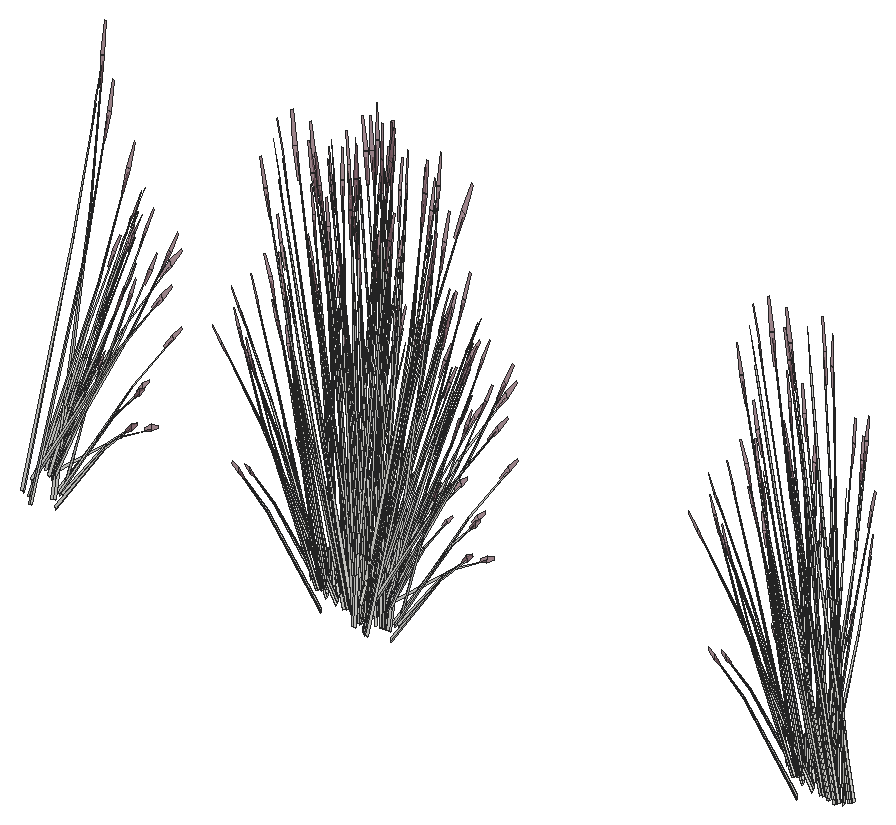
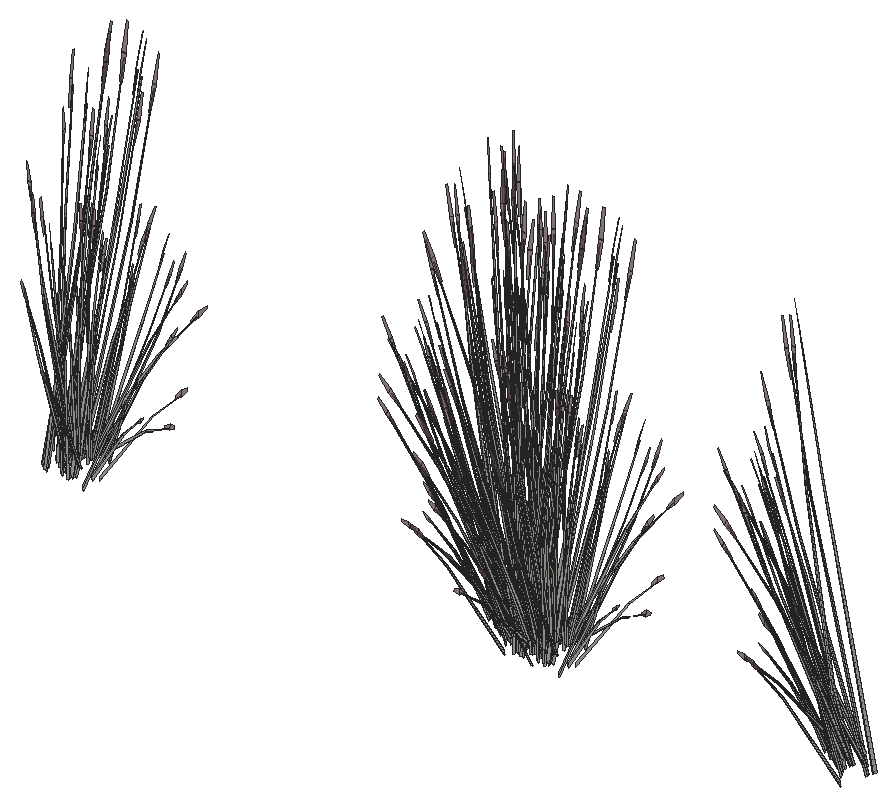
# SketchUp Ruby script. Lengths in inches.
U = 1.inch
M = Sketchup.active_model
def pt(a) = Geom::Point3d.new(a.map { |v| v * U })
def face(e, loops, mat)
  f = e.add_face(loops[0].map { |a| pt(a) })
  loops[1..].each { |l| e.add_face(l.map { |a| pt(a) }).erase! }
  f.material = f.back_material = mat if mat
  f
end
# faces: each face lists its corners as indices into pts; further lists are holes
def faces(e, pts, list, mat = nil) = list.each { |f| face(e, (f[0].is_a?(Array) ? f : [f]).map { |l| l.map { |i| pts[i] } }, mat) }
# xy, xz, yz: faces in a plane at the given z, y or x. An outline is a flat list of corners, or four numbers for a rectangle; further outlines are holes
def ring(l) = l.size == 4 ? [[l[0], l[1]], [l[2], l[1]], [l[2], l[3]], [l[0], l[3]]] : l.each_slice(2).to_a
def flat(e, list, mat, &to3) = list.each { |f| face(e, (f[0].is_a?(Array) ? f : [f]).map { |l| ring(l).map { |u, v| to3.(u, v) } }, mat) }
def xy(e, z, list, mat = nil) = flat(e, list, mat) { |x, y| [x, y, z] }
def xz(e, y, list, mat = nil) = flat(e, list, mat) { |x, z| [x, y, z] }
def yz(e, x, list, mat = nil) = flat(e, list, mat) { |y, z| [x, y, z] }
def lines(e, pts, list) = list.each { |a, b| e.add_line(pt(pts[a]), pt(pts[b])) }
# prism: a flat outline (further loops are holes) pulled along v
def prism(e, loops, v, mat = nil)
  f = face(e, loops, mat); d = Geom::Vector3d.new(v.map { |x| x * U })
  f.pushpull(f.normal.samedirection?(d) ? d.length : -d.length)
end
def box(e, o, s, mat = nil) = prism(e, [[o, [o[0] + s[0], o[1], o[2]], [o[0] + s[0], o[1] + s[1], o[2]], [o[0], o[1] + s[1], o[2]]]], [0, 0, s[2]], mat)
def at(x, y, z, deg = 0) = Geom::Transformation.translation(pt([x, y, z])) * Geom::Transformation.rotation(ORIGIN, Z_AXIS, deg.degrees)
def axes(o, x, y, z) = Geom::Transformation.new([*x, 0, *y, 0, *z, 0, *pt(o).to_a, 1])
def part(name) = M.definitions.add(name)
# library, detail: a bought-in or finely detailed component or shape, given as its bounding box
def library(name, o, s) = part(name).tap { |d| box(d.entities, o, s) }
def detail(e, o, s) = box(e.add_group.entities, o, s)
def put(e, d, t, mat = nil) = e.add_instance(d, t).tap { |i| i.material = mat if mat }
def group(e, t, mat = nil) = e.add_group.tap { |g| g.transformation = t; g.material = mat if mat }.entities
root = M.entities
M.materials.add("LightPink_Translucent").color = [144, 107, 117]
M.materials["LightPink_Translucent"].alpha = 0.75
c1 = part("blade")
p = [[2.15,0.21,22],[0,0.17,0],[0.09,0.45,0],[2.18,0.31,22],[2.29,0.31,22],[0.38,0.45,0],
  [2.48,0.24,33],[2.49,0.24,33],[2.48,0.22,33]]
faces(c1.entities,p,[[0,1,2,3],[4,5,2,3],[6,3,4,7],[8,0,3,6]])
c2 = part("seeds")
p = [[0.3,-0.1,1.38],[-0.01,-0.03,1.59],[-0.01,-0.03,0.03],[0.14,-0.07,-0.07],[0.29,-0.03,3],[0.15,0.01,3.11]]
faces(c2.entities,p,[[0,1,2,3],[1,0,4,5]],"LightPink_Translucent")
c3 = part("blade with seeds")
put(c3.entities,c1,at(0,0,0))
put(c3.entities,c2,axes([2.4,0.25,30.99],[1.5799,-0.05474,1.17369],[-0.12525,1.92788,0.29478],[-0.07173,-0.02425,1.56792]))
put(root,c3,axes([763.12,481.41,3.1875],[0.57465,0,0],[0,0.36542,-0.25804],[0,0.08323,0.81856]))
put(root,c3,axes([761.26,480.94,3.33],[0.46399,-0.21707,-0.14548],[0.30855,0.30672,-0.25001],[0.11448,0.03115,0.79854]))
put(root,c3,axes([762.375,482.77,3.33],[-0.2947,-0.01025,0.5253],[0.19462,-0.21779,0.29003],[0.11642,0.07737,0.41205]))
put(root,c3,axes([761.43,482.61,4.52],[0.27385,-0.27986,-0.0608],[0.39658,0.16123,-0.33747],[0.13785,0.07907,0.51278]))
put(root,c3,axes([761.75,482.47,4.34],[0.45348,-0.07772,-0.25549],[0.07933,0.29434,-0.1979],[0.1218,0.08435,0.48886]))
put(root,c3,axes([762.27,482.12,4.53],[-0.26148,-0.20471,0.17707],[0.29857,-0.19378,-0.2286],[0.1517,0.02948,0.4374]))
put(root,c3,axes([762.43,480.36,3.01],[0.4301,0.16348,-0.24825],[-0.25708,0.29314,0],[0.09796,0.03723,0.78752]))
put(root,c3,axes([762.51,482.3,4.37],[-0.02314,0.24862,0.03215],[-0.34943,-0.00682,0.2531],[0.13385,0.02602,0.38595]))
put(root,c3,axes([762.41,482.69,2.75],[0.03348,-0.0472,0.88171],[0.42153,-0.13902,-0.1347],[0.12779,0.07195,0.15018]))
put(root,c3,axes([762.54,482.22,4.37],[-0.33886,0.21544,0.24001],[-0.29224,-0.22879,0.1979],[0.15898,0.03974,0.49665]))
put(root,c3,axes([763.42,482.26,3.96],[-0.08796,-0.27485,-0.01746],[0.41573,-0.06319,-0.07916],[0.08682,0.01742,0.26109]))
put(root,c3,axes([761.8,480.99,3.03],[0.47805,0.0536,-0.31177],[-0.10088,0.33065,-0.08182],[0.14266,0.04007,0.68817]))
put(root,c3,axes([761.7,481.7,3.9375],[-0.1707,-0.05633,0.85688],[0.35326,-0.23632,0.06928],[0.22018,0.10661,0.36631]))
put(root,c3,axes([763.05,481.625,4.37],[0.16879,0.22293,0.03215],[-0.30779,0.10912,0.2531],[0.13568,-0.02153,0.38595]))
put(root,c3,axes([762.64,482.22,4.26],[0.26148,0.20471,-0.17707],[-0.29857,0.19378,0.2286],[0.1517,0.02948,0.4374]))
put(root,c3,axes([762.34,482.25,4.52],[0.02461,-0.33251,-0.0608],[0.4659,0.00909,-0.33747],[0.17944,0.0231,0.51278]))
put(root,c3,axes([763.01,481.55,4.37],[-0.12984,0.29812,0.24001],[-0.42685,-0.10194,0.1979],[0.16786,-0.01792,0.49665]))
put(root,c3,axes([762.75,482.05,4.36],[0.09858,-0.00553,0.87472],[0.2704,-0.25401,-0.13834],[0.17535,0.03353,0.07015]))
put(root,c3,axes([763.91,481.57,3.38],[-0.28394,0.05398,0.5743],[0.13365,-0.22308,0.42196],[0.15063,0.01526,0.12649]))
put(root,c3,axes([763.1,481.51,4.26],[0.38192,0.09121,-0.17707],[-0.11139,0.2661,0.2286],[0.15377,-0.0244,0.4374]))
put(root,c3,axes([762.37,482.09,4.49],[0.45939,0.00787,-0.35523],[-0.03085,0.3315,0.04287],[0.19462,0.03498,0.5025]))
put(root,c3,axes([763.62,481.26,2.75],[-0.02402,-0.04964,0.88171],[0.16658,-0.29036,-0.1347],[0.16804,-0.00418,0.15018]))
put(root,c3,axes([763.78,482.51,4.35],[-0.04155,-0.02862,0.88692],[0.0909,-0.30682,-0.08381],[0.16368,-0.0196,0.15695]))
put(root,c3,axes([762.0625,481.18,3.9375],[-0.19062,0.00741,0.85688],[0.12645,-0.32094,0.06928],[0.27165,0.01985,0.36631]))
put(root,c3,axes([763.38,481.93,3.3],[-0.11068,-0.08041,0.71501],[0.144,-0.26601,-0.15377],[0.22393,0.03604,0.3057]))
put(root,c3,axes([782.62,481.38,3.9375],[0.15946,-0.06916,0.85688],[0.13424,0.31957,0.06928],[-0.25033,0.07223,0.36631]))
put(root,c3,axes([782.125,481.92,3.3],[0.15971,0.02684,0.71501],[0.10294,0.27415,-0.15377],[-0.21694,0.05132,0.3057]))
put(root,c3,axes([783.54,481.05,3.67],[0.13063,-0.0473,0.88532],[0.04505,0.33024,0.06928],[-0.28294,0.04382,0.31642]))
put(root,c3,axes([782.13,481.27,4.36],[-0.07505,0.04245,0.87472],[0.00638,0.31015,-0.13834],[-0.17202,0.04033,0.07015]))
put(root,c3,axes([782.375,481.09,4.26],[-0.38192,-0.09121,-0.17707],[0.11139,-0.2661,0.2286],[-0.15377,0.0244,0.4374]))
put(root,c3,axes([781.3,481.58,4.35],[0.05865,0.00877,0.88692],[0.18143,0.28888,-0.08381],[-0.12006,0.07582,0.15695]))
put(root,c3,axes([782.64,481.23,4.34],[-0.1245,0.29741,-0.25549],[-0.42685,-0.10194,-0.1979],[-0.17186,0.02727,0.48886]))
put(root,c3,axes([782.42,481.21,2.75],[0.01165,0.05153,0.88171],[-0.23495,0.26909,-0.1347],[-0.16689,-0.01356,0.15018]))
put(root,c3,axes([781.79,482.5,3.38],[0.19152,-0.14818,0.5743],[0.07557,0.23459,0.42196],[-0.13841,0.042,0.12649]))
put(root,c3,axes([782.62,480.97,4.52],[0.23123,0.29606,-0.0608],[-0.41039,0.14549,-0.33747],[-0.17294,0.03906,0.51278]))
put(root,c3,axes([782.43,480.98,4.37],[-0.16879,-0.22293,0.03215],[0.30779,-0.10912,0.2531],[-0.13568,0.02153,0.38595]))
put(root,c3,axes([783.21,481.59,3.9375],[0.11478,-0.10046,0.85688],[0.28982,0.27117,0.06928],[-0.19878,0.12349,0.36631]))
put(root,c3,axes([782.52,481.86,4.26],[-0.40003,0.04673,-0.17707],[-0.10563,-0.26712,0.2286],[-0.11464,0.07175,0.4374]))
put(root,c3,axes([782.3,482.65,2.75],[0.06164,0.03267,0.88171],[0.10452,0.30266,-0.1347],[-0.13662,0.06454,0.15018]))
put(root,c3,axes([782.57,481.8,4.37],[-0.11397,-0.30091,0.24001],[0.44709,-0.05222,0.1979],[-0.13177,0.07077,0.49665]))
put(root,c3,axes([782.48,481.74,4.37],[-0.31549,-0.13751,0.03215],[0.18368,-0.19581,0.2531],[-0.10115,0.06331,0.38595]))
put(root,c3,axes([783.12,481.84,3.9375],[0.08557,-0.11238,0.85688],[0.35897,0.23257,0.06928],[-0.16194,0.14495,0.36631]))
put(root,c3,axes([782.78,481.06,4.53],[0.38192,0.09121,0.17707],[-0.11139,0.2661,-0.2286],[-0.15377,0.0244,0.4374]))
put(root,c3,axes([782.85,481.89,4.34],[0.11806,0.29854,-0.25549],[-0.44709,0.05222,-0.1979],[-0.12812,0.08019,0.48886]))
put(root,c3,axes([782.15,482.42,4.36],[-0.01142,0.0647,0.87472],[0.32418,0.22509,-0.13834],[-0.08487,0.10644,0.07015]))
put(root,c3,axes([783.33,482.3,3.01],[-0.4301,-0.16348,-0.24825],[0.25708,-0.29314,0],[-0.09796,-0.03723,0.78752]))
put(root,c3,axes([782.63,481.67,4.52],[0.4251,0.18028,-0.0608],[-0.24491,0.26108,-0.33747],[-0.1201,0.09075,0.51278]))
put(root,c3,axes([783.59,482.5,3.1875],[-0.28732,0.32763,0],[-0.4807,-0.18271,-0.25804],[-0.10948,-0.04161,0.81856]))
put(root,c3,axes([781.93,482.46,4.82],[0.40553,0.08728,-0.03244],[-0.12475,0.26862,-0.14708],[-0.06633,0.04078,0.48512]))
put(root,c3,axes([782.84,481.7,4.53],[0.40003,-0.04673,0.17707],[0.10563,0.26712,-0.2286],[-0.11464,0.07175,0.4374]))
put(root,c3,axes([783.07,482.97,3.3],[0.14502,-0.05158,0.71501],[0.35805,0.15552,-0.15377],[-0.10657,0.13457,0.3057]))
put(root,c3,axes([784.5,481.72,3.33],[-0.46399,0.21707,-0.14548],[-0.30855,-0.30672,-0.25001],[-0.11448,-0.03115,0.79854]))
put(root,c3,axes([783.22,482.41,4.37],[-0.32725,-0.22308,0.24001],[0.34753,-0.1924,0.1979],[-0.06036,0.10466,0.49665]))
put(root,c3,axes([783.45,482.18,3.01],[-0.10795,-0.28489,-0.15489],[0.42874,-0.0809,0.15489],[-0.08643,-0.03285,0.69487]))
put(root,c3,axes([783.1,482.39,4.37],[-0.37765,-0.01523,0.03215],[0.01035,-0.23004,0.2531],[-0.03952,0.08812,0.38595]))
put(root,c3,axes([783.22,482.48,4.26],[-0.31095,0.17214,-0.17707],[-0.29435,-0.19656,0.2286],[-0.04479,0.09987,0.4374]))
put(root,c3,axes([784.8125,481.96,3.03],[-0.30954,0.24575,-0.31177],[-0.38452,-0.22284,-0.08182],[-0.12404,0.0613,0.68817]))
put(root,c3,axes([782.11,483.09,4.35],[0.05214,-0.01974,0.88692],[0.43092,0.1313,-0.08381],[-0.01013,0.10932,0.15695]))
put(root,c3,axes([785.02,481.82,3.23],[-0.44875,-0.26316,-0.12596],[0.3776,-0.2955,0.27565],[-0.12084,0.03078,0.84108]))
put(root,c3,axes([783.43,482.29,4.67],[-0.01196,0.30243,-0.3943],[-0.50354,-0.02031,0.04758],[-0.05314,0.12813,0.55778]))
put(root,c3,axes([783.42,483.14,3.38],[-0.01189,-0.19441,0.5743],[0.29719,0.13866,0.42196],[-0.05845,0.09266,0.12649]))
put(root,c3,axes([784.8,481.77,3.11],[-0.49904,0.02018,-0.2237],[-0.04513,-0.33504,0.10766],[-0.08934,0.03396,0.71822]))
put(root,c3,axes([783.84,482.33,3.24],[0.4301,0.16348,0.24825],[-0.25708,0.29314,0],[-0.09796,-0.03723,0.78752]))
put(root,c3,axes([783.26,482.72,3.68],[0.0101,-0.16879,0.77173],[0.45413,0.08915,0.10664],[-0.03935,0.17989,0.36441]))
put(root,c3,axes([784.46,481.82,3.31],[-0.08866,0.29179,0.0724],[-0.43315,-0.05065,-0.20674],[-0.07883,-0.02996,0.63372]))
put(root,c3,axes([785.32,482.63,3.01],[-0.4301,0.16348,-0.24825],[-0.25708,-0.29314,0],[-0.09796,0.03723,0.78752]))
put(root,c3,axes([785.35,482.54,3.1],[-0.28374,-0.32877,-0.02571],[0.4807,-0.18271,0.25804],[-0.11845,0.0313,0.81815]))
put(root,c3,axes([783.53,482.39,4.5],[0.32898,0.21969,-0.2836],[-0.34753,0.1924,-0.21967],[-0.05006,0.11162,0.54264]))
put(root,c3,axes([785.22,482.5,3.01],[-0.42874,-0.0809,-0.15489],[0.10795,-0.28489,0.15489],[-0.08643,0.03285,0.69487]))
put(root,c3,axes([783.38,482.23,4.53],[0.31095,-0.17214,0.17707],[0.29435,0.19656,-0.2286],[-0.04479,0.09987,0.4374]))
put(root,c3,axes([785.47,481.28,3.42],[-0.01255,-0.30784,0.70636],[0.56816,0.0798,0.29908],[-0.13438,0.16845,0.66675]))
put(root,c3,axes([783.18,482.28,4.7],[0.50507,0.0162,-0.06749],[-0.01381,0.30672,-0.3746],[-0.03508,0.11813,0.56919]))
put(root,c3,axes([783.17,482.72,3.41],[0.41748,-0.0579,0.03254],[0.09598,0.23326,-0.43152],[-0.02647,0.11808,0.3868]))
put(root,c3,axes([785.15,481.68,3.33],[0.05355,0.37308,-0.14548],[-0.55775,0.02256,-0.25001],[-0.09822,0.04969,0.79854]))
put(root,c3,axes([783.9,482.08,3.9375],[-0.01125,-0.12549,0.85688],[0.48751,0.08325,0.06928],[-0.03015,0.17883,0.36631]))
put(root,c3,axes([784.32,481.54,3.18],[0.58084,0.06889,0.22877],[-0.11821,0.38906,0.08977],[-0.08488,-0.03757,0.79428]))
put(root,c3,axes([784,482.16,3.24],[0.49383,-0.08678,0.08821],[0.12194,0.32295,0.17543],[-0.04404,-0.04705,0.80203]))
put(root,c3,axes([784.64,482.21,3.1],[-0.4633,-0.14679,0],[0.22297,-0.30501,0],[0,0,0.81353]))
put(root,c3,axes([785.71,482.58,3.1875],[0.28732,0.32763,0],[-0.4807,0.18271,-0.25804],[-0.10948,0.04161,0.81856]))
put(root,c3,axes([784.25,482.72,4.53],[-0.45283,-0.08548,0.26641],[0.15485,-0.28101,0.21967],[0.02721,0.11051,0.55128]))
put(root,c3,axes([784.13,482.74,4.37],[-0.33863,0.11112,0.03215],[-0.16575,-0.20263,0.2531],[0.0327,0.08932,0.38595]))
put(root,c3,axes([785.47,482.18,3.24],[0.13276,-0.32494,0.08821],[0.4858,0.09195,0.17543],[-0.08392,0.00158,0.80203]))
put(root,c3,axes([785.25,481.75,3.31],[0.33952,0.19644,0.0724],[-0.2832,0.22163,-0.20674],[-0.07883,0.02996,0.63372]))
put(root,c3,axes([785.24,481.6,3.36],[0.49904,-0.02018,0.2237],[0.04513,0.33504,-0.10766],[-0.08934,0.03396,0.71822]))
put(root,c3,axes([785.36,482.375,3.17],[0.57533,0.10627,0.15378],[-0.14394,0.37986,-0.18246],[-0.09522,0.04754,0.82443]))
put(root,c3,axes([785.61,482.35,3.24],[0.4301,-0.16348,0.24825],[0.25708,0.29314,0],[-0.09796,0.03723,0.78752]))
put(root,c3,axes([784.74,482.09,3.1],[-0.14994,-0.28188,0],[0.42817,-0.09871,0],[0,0,0.77185]))
put(root,c3,axes([784.2,482.68,2.75],[0.07437,-0.01779,0.88171],[0.44738,0.09793,-0.1347],[0.01308,0.11037,0.15018]))
put(root,c3,axes([784.3,482.78,4.26],[-0.13855,0.25143,-0.17707],[-0.4042,-0.07334,0.2286],[0.03706,0.10123,0.4374]))
put(root,c3,axes([785.35,481.53,3.11],[-0.22297,0.29461,-0.2237],[-0.4633,-0.14179,0.10766],[0,0.06791,0.71822]))
put(root,c3,axes([784.01,483.23,4.36],[0.05825,0.05265,0.87472],[0.47011,0.02068,-0.13834],[0.04727,0.11612,0.07015]))
put(root,c3,axes([786.23,481.35,3.24],[-0.36107,-0.23816,0.08821],[0.36387,-0.231,0.17543],[-0.03988,0.04864,0.80203]))
put(root,c3,axes([785.27,481.36,3.15],[0,0.37813,-0.02818],[-0.57465,0,0],[0,0.01188,0.89684]))
put(root,c3,axes([784.25,482.51,4.53],[0.13855,-0.25143,0.17707],[0.4042,0.07334,-0.2286],[0.03706,0.10123,0.4374]))
put(root,c3,axes([785,482.1,3.15],[0.1998,0.37562,-0.03006],[-0.5709,0.13162,0],[0.00698,0.01312,0.86086]))
put(root,c3,axes([784.34,482.55,4.49],[0.21934,0.26585,-0.35523],[-0.45151,0.14816,0.04287],[0.05129,0.12845,0.5025]))
put(root,c3,axes([786.65,481.6,3.1],[-0.57436,-0.00261,-0.02488],[0,-0.36542,0.24971],[-0.01805,0.08319,0.79176]))
put(root,c3,axes([785.52,480.5,3.24],[-0.49383,0.08678,0.08821],[-0.12194,-0.32295,0.17543],[0.04404,0.04705,0.80203]))
put(root,c3,axes([784.8,483.41,4.82],[0.31757,-0.18757,-0.03244],[0.29098,0.20543,-0.14708],[0.02049,0.05821,0.48512]))
put(root,c3,axes([785.36,481.44,3.11],[0.32079,0.21119,0],[-0.32079,0.21119,0],[0,0,0.84633]))
put(root,c3,axes([785.36,481.19,3.36],[0.22297,-0.29461,0.2237],[0.4633,0.14179,-0.10766],[0,0.06791,0.71822]))
put(root,c3,axes([785.16,482.22,3.1],[0.4633,0.14679,0],[-0.22297,0.30501,0],[0,0,0.87477]))
put(root,c3,axes([784.5,482.61,4.34],[0.45175,0.08196,-0.25549],[-0.15485,0.28101,-0.1979],[0.04142,0.11314,0.48886]))
put(root,c3,axes([784.12,482.62,4.52],[0.44971,-0.15222,-0.0608],[0.221,0.27017,-0.33747],[0.05933,0.11385,0.51278]))
put(root,c3,axes([785.21,481.125,3.19],[-0.58084,-0.06889,0.24599],[0.11821,-0.38906,0.09653],[0.08488,0.03757,0.85407]))
put(root,c3,axes([786.53,481.66,3.01],[-0.32079,0.20399,-0.15489],[-0.32079,-0.20399,0.15489],[0,0.06571,0.69487]))
put(root,c3,axes([785.61,481.62,3.05],[0.16851,0.29936,-0.34606],[-0.4854,0.10781,-0.09083],[0.01863,0.10137,0.76386]))
put(root,c3,axes([785.375,481.3,3.1],[0.51416,0,0],[0,0.33849,0],[0,0,0.89203]))
put(root,c3,axes([784.88,480.92,3.36],[-0.27607,-0.27443,0.2237],[0.41817,-0.19325,-0.10766],[0.08934,0.03396,0.71822]))
put(root,c3,axes([785.55,481.26,3.31],[0.42817,-0.09535,0.0724],[0.14994,0.27228,-0.20674],[0,0.05992,0.63372]))
put(root,c3,axes([785.41,481.28,3.33],[0.51755,0.15601,-0.14548],[-0.2492,0.32927,-0.25001],[0.01626,0.08084,0.79854]))
put(root,c3,axes([786.53,481.36,3.24],[0,-0.32696,0.24825],[0.51416,0,0],[0,0.07447,0.78752]))
put(root,c3,axes([786.75,481.66,3.01],[0,0.32696,-0.24825],[-0.51416,0,0],[0,0.07447,0.78752]))
put(root,c3,axes([785.375,482.65,4.37],[-0.45708,0.07503,0.24001],[-0.07933,-0.29434,0.1979],[0.1075,0.08675,0.49665]))
put(root,c3,axes([785.29,482.71,4.37],[-0.20887,0.2077,0.03215],[-0.29744,-0.12092,0.2531],[0.09616,0.06659,0.38595]))
put(root,c3,axes([784.76,482.03,3.9375],[-0.10505,-0.10498,0.85688],[0.48542,-0.08838,0.06928],[0.10971,0.1648,0.36631]))
put(root,c3,axes([785.31,482.05,3.09],[0.48247,-0.11094,-0.09599],[0.16954,0.31956,0.00004],[0.05326,-0.01226,0.86949]))
put(root,c3,axes([785.22,482.47,4.53],[-0.07098,-0.26335,0.17707],[0.40574,-0.06954,-0.2286],[0.10898,0.07547,0.4374]))
put(root,c3,axes([785.31,481.1,3.11],[0.27607,0.27443,-0.2237],[-0.41817,0.19325,0.10766],[0.08934,0.03396,0.71822]))
put(root,c3,axes([785.5,480.96,4.24],[-0.39711,-0.16988,0.69141],[0.41931,-0.2645,0.29833],[0.12812,0.1594,0.66832]))
put(root,c3,axes([784.83,482.84,4.35],[0.00136,-0.03958,0.88692],[0.39383,-0.17464,-0.08381],[0.1368,0.06234,0.15695]))
put(root,c3,axes([786.1,482.34,3.38],[-0.25875,-0.09401,0.5743],[0.33411,-0.09552,0.42196],[0.09012,0.08091,0.12649]))
put(root,c3,axes([785.18,482.24,3.3],[0.00811,-0.10838,0.71501],[0.38755,-0.12106,-0.15377],[0.11964,0.12972,0.3057]))
put(root,c3,axes([786.07,480.49,3.01],[0.10795,0.28489,-0.15489],[-0.42874,0.0809,0.15489],[0.08643,0.03285,0.69487]))
put(root,c3,axes([786.88,481.41,3.1875],[0.57465,0,0],[0,0.36542,-0.25804],[0,0.08323,0.81856]))
put(root,c3,axes([785.02,480.94,3.33],[0.46399,-0.21707,-0.14548],[0.30855,0.30672,-0.25001],[0.11448,0.03115,0.79854]))
put(root,c3,axes([786.14,482.77,3.33],[-0.2947,-0.01025,0.5253],[0.19462,-0.21779,0.29003],[0.11642,0.07737,0.41205]))
put(root,c3,axes([785.1875,482.61,4.52],[0.27385,-0.27986,-0.0608],[0.39658,0.16123,-0.33747],[0.13785,0.07907,0.51278]))
put(root,c3,axes([785.51,482.47,4.34],[0.45348,-0.07772,-0.25549],[0.07933,0.29434,-0.1979],[0.1218,0.08435,0.48886]))
put(root,c3,axes([786.03,482.12,4.53],[-0.26148,-0.20471,0.17707],[0.29857,-0.19378,-0.2286],[0.1517,0.02948,0.4374]))
put(root,c3,axes([786.19,480.36,3.01],[0.4301,0.16348,-0.24825],[-0.25708,0.29314,0],[0.09796,0.03723,0.78752]))
put(root,c3,axes([786.27,482.3,4.37],[-0.02314,0.24862,0.03215],[-0.34943,-0.00682,0.2531],[0.13385,0.02602,0.38595]))
put(root,c3,axes([786.17,482.69,2.75],[0.03348,-0.0472,0.88171],[0.42153,-0.13902,-0.1347],[0.12779,0.07195,0.15018]))
put(root,c3,axes([786.3,482.22,4.37],[-0.33886,0.21544,0.24001],[-0.29224,-0.22879,0.1979],[0.15898,0.03974,0.49665]))
put(root,c3,axes([787.18,482.26,3.96],[-0.08796,-0.27485,-0.01746],[0.41573,-0.06319,-0.07916],[0.08682,0.01742,0.26109]))
put(root,c3,axes([785.5625,480.99,3.03],[0.47805,0.0536,-0.31177],[-0.10088,0.33065,-0.08182],[0.14266,0.04007,0.68817]))
put(root,c3,axes([785.46,481.7,3.9375],[-0.1707,-0.05633,0.85688],[0.35326,-0.23632,0.06928],[0.22018,0.10661,0.36631]))
put(root,c3,axes([786.81,481.625,4.37],[0.16879,0.22293,0.03215],[-0.30779,0.10912,0.2531],[0.13568,-0.02153,0.38595]))
put(root,c3,axes([786.4,482.22,4.26],[0.26148,0.20471,-0.17707],[-0.29857,0.19378,0.2286],[0.1517,0.02948,0.4374]))
put(root,c3,axes([786.1,482.25,4.52],[0.02461,-0.33251,-0.0608],[0.4659,0.00909,-0.33747],[0.17944,0.0231,0.51278]))
put(root,c3,axes([786.78,481.55,4.37],[-0.12984,0.29812,0.24001],[-0.42685,-0.10194,0.1979],[0.16786,-0.01792,0.49665]))
put(root,c3,axes([786.51,482.05,4.36],[0.09858,-0.00553,0.87472],[0.2704,-0.25401,-0.13834],[0.17535,0.03353,0.07015]))
put(root,c3,axes([787.68,481.57,3.38],[-0.28394,0.05398,0.5743],[0.13365,-0.22308,0.42196],[0.15063,0.01526,0.12649]))
put(root,c3,axes([786.87,481.51,4.26],[0.38192,0.09121,-0.17707],[-0.11139,0.2661,0.2286],[0.15377,-0.0244,0.4374]))
put(root,c3,axes([786.13,482.09,4.49],[0.45939,0.00787,-0.35523],[-0.03085,0.3315,0.04287],[0.19462,0.03498,0.5025]))
put(root,c3,axes([787.38,481.26,2.75],[-0.02402,-0.04964,0.88171],[0.16658,-0.29036,-0.1347],[0.16804,-0.00418,0.15018]))
put(root,c3,axes([787.54,482.51,4.35],[-0.04155,-0.02862,0.88692],[0.0909,-0.30682,-0.08381],[0.16368,-0.0196,0.15695]))
put(root,c3,axes([785.82,481.18,3.9375],[-0.19062,0.00741,0.85688],[0.12645,-0.32094,0.06928],[0.27165,0.01985,0.36631]))
put(root,c3,axes([787.14,481.93,3.3],[-0.11068,-0.08041,0.71501],[0.144,-0.26601,-0.15377],[0.22393,0.03604,0.3057]))
put(root,c3,axes([816.32,481.38,3.9375],[0.15946,-0.06916,0.85688],[0.13424,0.31957,0.06928],[-0.25033,0.07223,0.36631]))
put(root,c3,axes([815.82,481.92,3.3],[0.15971,0.02684,0.71501],[0.10294,0.27415,-0.15377],[-0.21694,0.05132,0.3057]))
put(root,c3,axes([817.23,481.05,3.67],[0.13063,-0.0473,0.88532],[0.04505,0.33024,0.06928],[-0.28294,0.04382,0.31642]))
put(root,c3,axes([815.83,481.27,4.36],[-0.07505,0.04245,0.87472],[0.00638,0.31015,-0.13834],[-0.17202,0.04033,0.07015]))
put(root,c3,axes([816.07,481.09,4.26],[-0.38192,-0.09121,-0.17707],[0.11139,-0.2661,0.2286],[-0.15377,0.0244,0.4374]))
put(root,c3,axes([815,481.58,4.35],[0.05865,0.00877,0.88692],[0.18143,0.28888,-0.08381],[-0.12006,0.07582,0.15695]))
put(root,c3,axes([816.33,481.23,4.34],[-0.1245,0.29741,-0.25549],[-0.42685,-0.10194,-0.1979],[-0.17186,0.02727,0.48886]))
put(root,c3,axes([816.12,481.21,2.75],[0.01165,0.05153,0.88171],[-0.23495,0.26909,-0.1347],[-0.16689,-0.01356,0.15018]))
put(root,c3,axes([815.49,482.5,3.38],[0.19152,-0.14818,0.5743],[0.07557,0.23459,0.42196],[-0.13841,0.042,0.12649]))
put(root,c3,axes([816.3125,480.97,4.52],[0.23123,0.29606,-0.0608],[-0.41039,0.14549,-0.33747],[-0.17294,0.03906,0.51278]))
put(root,c3,axes([816.13,480.98,4.37],[-0.16879,-0.22293,0.03215],[0.30779,-0.10912,0.2531],[-0.13568,0.02153,0.38595]))
put(root,c3,axes([816.9,481.59,3.9375],[0.11478,-0.10046,0.85688],[0.28982,0.27117,0.06928],[-0.19878,0.12349,0.36631]))
put(root,c3,axes([816.21,481.86,4.26],[-0.40003,0.04673,-0.17707],[-0.10563,-0.26712,0.2286],[-0.11464,0.07175,0.4374]))
put(root,c3,axes([815.99,482.65,2.75],[0.06164,0.03267,0.88171],[0.10452,0.30266,-0.1347],[-0.13662,0.06454,0.15018]))
put(root,c3,axes([816.26,481.8,4.37],[-0.11397,-0.30091,0.24001],[0.44709,-0.05222,0.1979],[-0.13177,0.07077,0.49665]))
put(root,c3,axes([816.17,481.74,4.37],[-0.31549,-0.13751,0.03215],[0.18368,-0.19581,0.2531],[-0.10115,0.06331,0.38595]))
put(root,c3,axes([816.82,481.84,3.9375],[0.08557,-0.11238,0.85688],[0.35897,0.23257,0.06928],[-0.16194,0.14495,0.36631]))
put(root,c3,axes([816.47,481.06,4.53],[0.38192,0.09121,0.17707],[-0.11139,0.2661,-0.2286],[-0.15377,0.0244,0.4374]))
put(root,c3,axes([816.54,481.89,4.34],[0.11806,0.29854,-0.25549],[-0.44709,0.05222,-0.1979],[-0.12812,0.08019,0.48886]))
put(root,c3,axes([815.84,482.42,4.36],[-0.01142,0.0647,0.87472],[0.32418,0.22509,-0.13834],[-0.08487,0.10644,0.07015]))
put(root,c3,axes([817.03,482.3,3.01],[-0.4301,-0.16348,-0.24825],[0.25708,-0.29314,0],[-0.09796,-0.03723,0.78752]))
put(root,c3,axes([816.33,481.67,4.52],[0.4251,0.18028,-0.0608],[-0.24491,0.26108,-0.33747],[-0.1201,0.09075,0.51278]))
put(root,c3,axes([817.29,482.5,3.1875],[-0.28732,0.32763,0],[-0.4807,-0.18271,-0.25804],[-0.10948,-0.04161,0.81856]))
put(root,c3,axes([815.63,482.46,4.82],[0.40553,0.08728,-0.03244],[-0.12475,0.26862,-0.14708],[-0.06633,0.04078,0.48512]))
put(root,c3,axes([816.54,481.7,4.53],[0.40003,-0.04673,0.17707],[0.10563,0.26712,-0.2286],[-0.11464,0.07175,0.4374]))
put(root,c3,axes([816.77,482.97,3.3],[0.14502,-0.05158,0.71501],[0.35805,0.15552,-0.15377],[-0.10657,0.13457,0.3057]))
put(root,c3,axes([818.2,481.72,3.33],[-0.46399,0.21707,-0.14548],[-0.30855,-0.30672,-0.25001],[-0.11448,-0.03115,0.79854]))
put(root,c3,axes([816.92,482.41,4.37],[-0.32725,-0.22308,0.24001],[0.34753,-0.1924,0.1979],[-0.06036,0.10466,0.49665]))
put(root,c3,axes([817.15,482.18,3.01],[-0.10795,-0.28489,-0.15489],[0.42874,-0.0809,0.15489],[-0.08643,-0.03285,0.69487]))
put(root,c3,axes([816.8,482.39,4.37],[-0.37765,-0.01523,0.03215],[0.01035,-0.23004,0.2531],[-0.03952,0.08812,0.38595]))
put(root,c3,axes([816.91,482.48,4.26],[-0.31095,0.17214,-0.17707],[-0.29435,-0.19656,0.2286],[-0.04479,0.09987,0.4374]))
put(root,c3,axes([818.51,481.96,3.03],[-0.30954,0.24575,-0.31177],[-0.38452,-0.22284,-0.08182],[-0.12404,0.0613,0.68817]))
put(root,c3,axes([815.81,483.09,4.35],[0.05214,-0.01974,0.88692],[0.43092,0.1313,-0.08381],[-0.01013,0.10932,0.15695]))
put(root,c3,axes([818.72,481.82,3.23],[-0.44875,-0.26316,-0.12596],[0.3776,-0.2955,0.27565],[-0.12084,0.03078,0.84108]))
put(root,c3,axes([817.12,482.29,4.67],[-0.01196,0.30243,-0.3943],[-0.50354,-0.02031,0.04758],[-0.05314,0.12813,0.55778]))
put(root,c3,axes([817.11,483.14,3.38],[-0.01189,-0.19441,0.5743],[0.29719,0.13866,0.42196],[-0.05845,0.09266,0.12649]))
put(root,c3,axes([818.49,481.77,3.11],[-0.49904,0.02018,-0.2237],[-0.04513,-0.33504,0.10766],[-0.08934,0.03396,0.71822]))
put(root,c3,axes([817.54,482.33,3.24],[0.4301,0.16348,0.24825],[-0.25708,0.29314,0],[-0.09796,-0.03723,0.78752]))
put(root,c3,axes([816.95,482.72,3.68],[0.0101,-0.16879,0.77173],[0.45413,0.08915,0.10664],[-0.03935,0.17989,0.36441]))
put(root,c3,axes([818.15,481.82,3.31],[-0.08866,0.29179,0.0724],[-0.43315,-0.05065,-0.20674],[-0.07883,-0.02996,0.63372]))
put(root,c3,axes([819.02,482.63,3.01],[-0.4301,0.16348,-0.24825],[-0.25708,-0.29314,0],[-0.09796,0.03723,0.78752]))
put(root,c3,axes([819.04,482.54,3.1],[-0.28374,-0.32877,-0.02571],[0.4807,-0.18271,0.25804],[-0.11845,0.0313,0.81815]))
put(root,c3,axes([817.22,482.39,4.5],[0.32898,0.21969,-0.2836],[-0.34753,0.1924,-0.21967],[-0.05006,0.11162,0.54264]))
put(root,c3,axes([818.91,482.5,3.01],[-0.42874,-0.0809,-0.15489],[0.10795,-0.28489,0.15489],[-0.08643,0.03285,0.69487]))
put(root,c3,axes([817.08,482.23,4.53],[0.31095,-0.17214,0.17707],[0.29435,0.19656,-0.2286],[-0.04479,0.09987,0.4374]))
put(root,c3,axes([819.16,481.28,3.42],[-0.01255,-0.30784,0.70636],[0.56816,0.0798,0.29908],[-0.13438,0.16845,0.66675]))
put(root,c3,axes([816.88,482.28,4.7],[0.50507,0.0162,-0.06749],[-0.01381,0.30672,-0.3746],[-0.03508,0.11813,0.56919]))
put(root,c3,axes([816.87,482.72,3.41],[0.41748,-0.0579,0.03254],[0.09598,0.23326,-0.43152],[-0.02647,0.11808,0.3868]))
put(root,c3,axes([818.84,481.68,3.33],[0.05355,0.37308,-0.14548],[-0.55775,0.02256,-0.25001],[-0.09822,0.04969,0.79854]))
